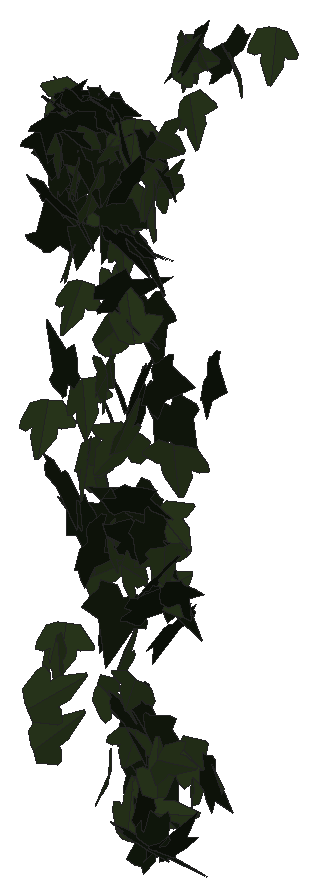
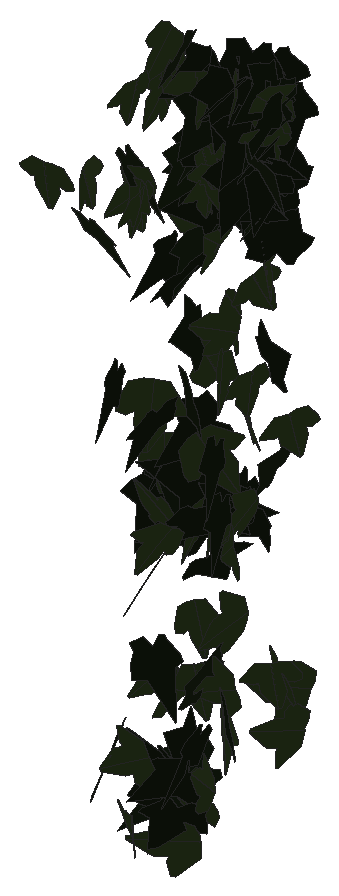
# SketchUp Ruby script. Lengths in inches.
U = 1.inch
M = Sketchup.active_model
def pt(a) = Geom::Point3d.new(a.map { |v| v * U })
def face(e, loops, mat)
  f = e.add_face(loops[0].map { |a| pt(a) })
  loops[1..].each { |l| e.add_face(l.map { |a| pt(a) }).erase! }
  f.material = f.back_material = mat if mat
  f
end
# faces: each face lists its corners as indices into pts; further lists are holes
def faces(e, pts, list, mat = nil) = list.each { |f| face(e, (f[0].is_a?(Array) ? f : [f]).map { |l| l.map { |i| pts[i] } }, mat) }
# xy, xz, yz: faces in a plane at the given z, y or x. An outline is a flat list of corners, or four numbers for a rectangle; further outlines are holes
def ring(l) = l.size == 4 ? [[l[0], l[1]], [l[2], l[1]], [l[2], l[3]], [l[0], l[3]]] : l.each_slice(2).to_a
def flat(e, list, mat, &to3) = list.each { |f| face(e, (f[0].is_a?(Array) ? f : [f]).map { |l| ring(l).map { |u, v| to3.(u, v) } }, mat) }
def xy(e, z, list, mat = nil) = flat(e, list, mat) { |x, y| [x, y, z] }
def xz(e, y, list, mat = nil) = flat(e, list, mat) { |x, z| [x, y, z] }
def yz(e, x, list, mat = nil) = flat(e, list, mat) { |y, z| [x, y, z] }
def lines(e, pts, list) = list.each { |a, b| e.add_line(pt(pts[a]), pt(pts[b])) }
# prism: a flat outline (further loops are holes) pulled along v
def prism(e, loops, v, mat = nil)
  f = face(e, loops, mat); d = Geom::Vector3d.new(v.map { |x| x * U })
  f.pushpull(f.normal.samedirection?(d) ? d.length : -d.length)
end
def box(e, o, s, mat = nil) = prism(e, [[o, [o[0] + s[0], o[1], o[2]], [o[0] + s[0], o[1] + s[1], o[2]], [o[0], o[1] + s[1], o[2]]]], [0, 0, s[2]], mat)
def at(x, y, z, deg = 0) = Geom::Transformation.translation(pt([x, y, z])) * Geom::Transformation.rotation(ORIGIN, Z_AXIS, deg.degrees)
def axes(o, x, y, z) = Geom::Transformation.new([*x, 0, *y, 0, *z, 0, *pt(o).to_a, 1])
def part(name) = M.definitions.add(name)
# library, detail: a bought-in or finely detailed component or shape, given as its bounding box
def library(name, o, s) = part(name).tap { |d| box(d.entities, o, s) }
def detail(e, o, s) = box(e.add_group.entities, o, s)
def put(e, d, t, mat = nil) = e.add_instance(d, t).tap { |i| i.material = mat if mat }
def group(e, t, mat = nil) = e.add_group.tap { |g| g.transformation = t; g.material = mat if mat }.entities
root = M.entities
M.materials.add("efeu1").color = [18, 25, 13]
M.materials.add("efeu2").color = [43, 57, 29]
c1 = part("ivyleaf_10")
p = [[0,0.5,-0.03],[-0.0625,2.02,-0.43],[-0.19,2.01,-0.46],[-0.54,1.05,-0.29],[-0.52,0.625,-0.18],[-0.83,0.76,-0.28],
  [-1.16,0.64,-0.33],[-1.15,0.33,-0.24],[-0.77,-0.39,0.02],[-0.3,-0.51,0.16],[0.04,-0.48,0.23],[-0.02,2.01,-0.4375],
  [-0.06,2.01,-0.43],[0.04,-0.49,0.23],[0.67,-0.49,0.14],[1.38,0.36,-0.2],[1.375,0.51,-0.24],[0.81,0.65,-0.19],
  [0.62,0.59,-0.15],[0.6,1.09,-0.28],[0.5,1.23,-0.31]]
faces(c1.entities,p,[[0,1,2,3,4,5,6,7,8,9,10],[11,12,0,13,14,15,16,17,18,19,20]],"efeu2")
c2 = part("ivyleaf_9")
p = [[1.54,2.16,1.25],[1.36,2.04,1.19],[-0.21,0.99,0.68],[-0.71,1.11,0.82],[-0.85,0.86,0.67],[-0.8,0.17,0.21],
  [-0.9,-0.01,0.1],[-0.67,-0.16,-0.02],[-0.08,-0.08,-0.05],[-0.03,-0.6,-0.4],[0.65,-0.88,-0.66],[0.83,-0.6,-0.49],
  [1.29,-0.42,-0.43],[1.8125,-0.07,-0.26],[1.21,0.44,0.15]]
faces(c2.entities,p,[[0,1,2,3,4,5,6,7,8,9,10,11,12,13,14]],"efeu1")
put(root,c1,axes([585.52,128.9,222.65],[-0.54212,-0.81235,-0.06265],[0.0387,0.04949,-0.97662],[0.81384,-0.54348,0.00471]))
put(root,c1,axes([578.94,128.14,213.07],[0.2301,0.27895,-1.14359],[0.75107,0.86242,0.36148],[0.90636,-0.78547,-0.00923]))
put(root,c2,axes([585.55,128.49,221.7],[-0.16843,0.93935,0.08399],[-0.01678,0.08232,-0.95433],[-0.94295,-0.16925,0.00198]))
put(root,c1,axes([583.87,128.9,215.3125],[-0.8398,-0.13492,0.40747],[-0.40406,-0.05358,-0.85051],[0.14482,-0.9319,-0.01009]))
put(root,c1,axes([584.26,129.4,240.45],[0.591,-0.3393,0.87922],[0.78325,-0.40029,-0.68097],[0.52408,0.98085,0.02624]))
put(root,c1,axes([583.77,128.875,233.49],[1.03176,0.22803,0.28353],[-0.27668,-0.06193,1.05665],[0.23628,-1.06821,-0.00074]))
put(root,c1,axes([580.61,129.42,225.9375],[0.68534,-0.54383,0.62493],[0.48946,-0.38853,-0.8749],[0.66836,0.84218,-0.00008]))
put(root,c2,axes([585.53,128.27,231.74],[0.19674,0.06037,-0.97596],[-0.53263,0.84148,-0.05532],[0.82003,0.53208,0.19823]))
put(root,c1,axes([582.47,128.65,210.42],[0.258,-0.77552,-0.70588],[-0.26578,0.65484,-0.81659],[1.01443,0.36881,-0.03442]))
put(root,c1,axes([579.13,128.17,211.02],[0.13674,0.28511,-1.14107],[0.52764,1.0118,0.31605],[1.05116,-0.54497,-0.0102]))
put(root,c2,axes([579.0625,129.56,224.1],[0.38561,-0.86651,0.45505],[0.21061,-0.40417,-0.9481],[0.9558,0.43864,0.02533]))
put(root,c1,axes([582.14,128.72,230.53],[0.60013,-0.50816,-0.7164],[-0.37655,0.63502,-0.76587],[0.79351,0.68566,0.17838]))
put(root,c2,axes([579.81,128.97,242.88],[0.24566,0.88942,-0.62998],[-0.19521,-0.59944,-0.92242],[-1.07231,0.31289,0.0236]))
put(root,c2,axes([582.44,129.68,218.75],[-0.31214,-1.02487,0.06024],[-0.01116,-0.05958,-1.07133],[1.02658,-0.31227,0.00667]))
put(root,c2,axes([582.68,128.41,234.93],[0.42243,0.24262,0.96228],[0.78221,0.56223,-0.48513],[-0.61074,0.88788,0.04424]))
put(root,c2,axes([583.09,128.75,238.09],[0.98483,0.26717,-0.34487],[-0.34553,-0.0421,-1.01933],[-0.26631,1.04262,0.04721]))
put(root,c2,axes([584.45,128.92,223.63],[0.54954,-0.67759,-0.64036],[-0.36194,0.52997,-0.87139],[0.85918,0.65665,0.0425]))
put(root,c1,axes([585.16,128.76,210.67],[0.07017,0.97933,-0.387],[-0.00979,0.38845,0.98122],[1.05298,-0.06165,0.03491]))
put(root,c1,axes([583.65,128.98,212.43],[0.85574,0.31412,-0.23921],[-0.34595,0.32134,-0.81563],[-0.19029,0.82841,0.40709]))
put(root,c1,axes([580.97,129.32,238.61],[0.13724,-1.08276,-0.04315],[0.03719,-0.03876,1.09095],[-1.08298,-0.13854,0.03199]))
put(root,c2,axes([584.12,128.51,219.38],[0.54084,0.38582,0.68539],[0.51903,0.44988,-0.66282],[-0.59095,0.74824,0.04511]))
put(root,c2,axes([581.52,128.47,221.9],[0.14842,-0.06138,-1.12897],[-0.78639,0.81252,-0.14756],[0.81236,0.79776,0.06342]))
put(root,c1,axes([582.93,129,227.37],[0.25347,-0.95085,0.36997],[-0.07167,0.36368,0.98378],[-1.01777,-0.26241,0.02287]))
put(root,c1,axes([580.34,129.04,240.625],[0.51319,-0.83155,-0.41195],[-0.09299,0.4223,-0.96828],[0.92332,0.50471,0.13145]))
put(root,c2,axes([585.04,128.85,207.48],[-0.86174,0.08361,-0.60119],[-0.59853,0.05649,0.86579],[0.1009,1.04921,0.0013]))
put(root,c1,axes([584.46,129.84,241.3],[0.17698,-0.79659,0.68255],[0.3458,-0.6092,-0.80066],[0.99038,0.35506,0.15759]))
put(root,c2,axes([583.84,128.58,207.7],[1.45844,-0.06622,-0.10201],[-0.07329,0.5011,-1.37309],[0.09706,1.37345,0.49605]))
put(root,c2,axes([579.14,129.06,241.66],[0.53688,0.79531,-0.56534],[-0.31461,-0.46971,-0.95956],[-0.92366,0.62227,-0.00176]))
put(root,c1,axes([585.58,128.85,212.04],[-0.26101,-0.39466,-0.79136],[0.44292,0.65581,-0.47315],[0.7654,-0.51409,0.00393]))
put(root,c2,axes([583.01,128.83,224.63],[0.8427,0.49196,0.32927],[0.29036,0.15569,-0.97572],[-0.51588,0.89125,-0.01131]))
put(root,c2,axes([583.47,128.53,241.17],[-0.21376,0.56597,-0.88787],[-0.3776,0.80452,0.60374],[0.98288,0.43217,0.03884]))
put(root,c2,axes([582.53,130.01,212.86],[0.33744,-0.86068,0.59164],[0.3391,-0.49778,-0.91755],[0.98783,0.46488,0.11287]))
put(root,c1,axes([579,129.68,241.5],[0.29646,-0.93548,0.17038],[0.23257,-0.10171,-0.96313],[0.92199,0.32646,0.18817]))
put(root,c2,axes([579.89,129.73,241.35],[0.49213,-0.9195,-0.04882],[-0.02424,0.0424,-1.04291],[0.92047,0.49272,-0.00136]))
put(root,c2,axes([583.23,129.73,237.63],[0.61706,-0.77703,0.18831],[0.13739,-0.13128,-0.99191],[0.78763,0.63166,0.0255]))
put(root,c2,axes([585.39,129.06,220.6875],[0.74433,0.61958,-0.12804],[-0.08391,-0.09929,-0.9682],[-0.62709,0.74871,-0.02243]))
put(root,c2,axes([582.78,129.4,222.02],[0.54904,-0.15476,0.95297],[0.94806,-0.12076,-0.56582],[0.18246,1.09317,0.0724]))
put(root,c2,axes([577.85,129.79,237.98],[0.52872,-0.4296,0.7182],[0.60121,-0.39598,-0.67945],[0.58217,0.7991,0.04941]))
put(root,c2,axes([584.97,129.41,206.8],[0.46852,0.91791,0.16625],[-0.09763,-0.13677,1.03028],[0.92772,-0.47796,0.02446]))
put(root,c1,axes([578.03,129.78,226.87],[0.54704,0.86913,-0.2398],[-0.13372,-0.19917,-1.02694],[-0.89163,0.5631,0.00689]))
put(root,c1,axes([578.37,130.04,214.75],[0.7305,-0.29535,0.69025],[0.63552,-0.26951,-0.7879],[0.39974,0.96822,-0.00876]))
put(root,c2,axes([584.11,129.1,208.58],[0.018,-0.22074,1.05801],[0.32906,1.00904,0.20492],[-1.02948,0.31867,0.084]))
put(root,c1,axes([579.86,129.73,241.99],[-0.93456,-0.22475,0.28094],[-0.27652,-0.05155,-0.9611],[0.23016,-0.97451,-0.01395]))
put(root,c1,axes([584.54,129.98,219.93],[0.62137,-0.23138,-0.81582],[0.78794,-0.21628,0.66148],[-0.31342,-1.00243,0.04559]))
put(root,c2,axes([583.14,129.29,233.71],[0.78131,0.34884,-0.6272],[-0.71739,0.35315,-0.69724],[-0.02048,0.93761,0.49596]))
put(root,c2,axes([579.62,130.18,222.32],[-0.39694,-0.04592,-0.95874],[0.94327,0.17331,-0.39883],[0.1776,-1.02309,-0.02453]))
put(root,c2,axes([579.37,129.5625,229.09],[0.0552,0.013,1.05977],[-0.5311,0.91869,0.01639],[-0.91718,-0.5312,0.05429]))
put(root,c2,axes([580.15,129.73,243.48],[0.74838,0.43766,-0.76082],[-0.68377,-0.33618,-0.86598],[-0.55033,1.01287,0.04132]))
put(root,c2,axes([583.04,129.33,237.51],[1.0056,0.36089,-0.16373],[-0.29156,0.3713,-0.97233],[-0.26841,0.94878,0.44279]))
put(root,c2,axes([583.57,130.3,242.5],[0.59373,-0.82559,0.0581],[0.02891,-0.05077,-1.0169],[0.82712,0.59441,-0.00616]))
put(root,c1,axes([579.46,130.33,233.27],[0.33452,0.81783,-0.44955],[-0.2388,-0.38665,-0.88109],[-0.90218,0.40559,0.06653]))
put(root,c1,axes([582.11,130.15,237.01],[0.08343,0.99386,-0.10781],[-0.01299,-0.1071,-0.99735],[-0.9996,0.08434,0.00397]))
put(root,c1,axes([579.9,130.18,228.4],[0.1988,1.03837,-0.09617],[-0.01793,-0.09448,-1.05723],[-1.04266,0.19961,-0.00016]))
put(root,c2,axes([581.85,130.65,238.63],[-0.71991,-0.68236,-0.17883],[0.11771,0.13572,-0.99175],[0.69551,-0.72926,-0.01725]))
put(root,c2,axes([581.47,130.14,221.74],[-0.32575,0.15785,1.01209],[-0.9123,0.43823,-0.36197],[-0.46578,-0.96871,0.00117]))
put(root,c2,axes([578.2,130.54,235.29],[0.78771,0.20273,0.63781],[-0.63522,-0.08367,0.8111],[0.21071,-1.01009,0.06083]))
put(root,c1,axes([580.96,130.3,213.24],[0.38495,-0.06136,0.95296],[0.94684,0.15797,-0.37231],[-0.12402,1.01556,0.11549]))
put(root,c1,axes([582.92,129.625,220.59],[-0.24828,0.62545,0.83654],[-0.36423,0.75403,-0.67186],[-0.97894,-0.43918,0.03781]))
put(root,c1,axes([582.54,130.19,206.96],[1.13403,-0.11412,0.10794],[-0.10741,0.01072,1.13975],[-0.11463,-1.1391,-0.00008]))
put(root,c1,axes([579.61,130.5,240.43],[-0.83811,-0.65835,0.06001],[-0.0405,-0.04559,-1.06571],[0.65984,-0.83902,0.01081]))
put(root,c1,axes([581.78,129.9,221.51],[-0.36671,0.6527,0.75917],[-0.4522,0.61334,-0.74575],[-0.89323,-0.57846,0.06587]))
put(root,c2,axes([581.11,130.89,242.29],[0.13969,-0.07753,-0.99855],[0.99934,-0.05626,0.14416],[-0.0666,-1.0067,0.06884]))
put(root,c1,axes([584.44,130.01,242.95],[-0.19559,-0.71341,-0.80037],[0.18191,0.7797,-0.73944],[1.05662,-0.26629,-0.02085]))
put(root,c1,axes([578.36,130.63,215.2],[0.78528,0.64052,-0.09761],[-0.07543,-0.06196,-1.01338],[-0.64351,0.78889,-0.00034]))
put(root,c2,axes([580.72,131.11,241.02],[-0.28691,-0.95809,-0.03676],[0.0429,0.0255,-0.99956],[0.95784,-0.28813,0.03376]))
put(root,c1,axes([578.22,131.27,242.61],[-0.4296,-0.52454,0.73994],[0.04439,-0.82993,-0.56256],[0.90592,-0.20808,0.37846]))
put(root,c1,axes([578.84,130.55,235.07],[0.47019,-0.86818,-0.31057],[-0.11266,0.29192,-0.98659],[0.91515,0.48199,0.03811]))
put(root,c1,axes([581.21,130.69,237.85],[0.93812,0.34984,-0.01559],[-0.0324,0.04231,-0.99993],[-0.34868,0.9373,0.05095]))
put(root,c2,axes([582.97,129.85,229.22],[0.12675,0.21286,1.05108],[0.17479,1.04015,-0.23172],[-1.05808,0.19732,0.08764]))
put(root,c1,axes([581.72,130,234.1],[0.15099,0.60151,-0.79965],[-0.03363,0.81129,0.60392],[1.00006,-0.06354,0.14104]))
put(root,c2,axes([577.9,130.55,242.29],[0.87475,-0.32857,0.32868],[0.38241,0.11076,-0.90701],[0.26411,0.92787,0.22466]))
put(root,c1,axes([578.375,130.97,242.04],[0.99941,-0.12496,0.14333],[0.14086,-0.02865,-1.00714],[0.12775,1.00923,-0.01084]))
put(root,c1,axes([581.92,130.84,239.2],[0.97935,0.01814,-0.22956],[-0.22841,0.20366,-0.95838],[0.02919,0.98506,0.20237]))
put(root,c2,axes([578.48,130.0625,242.61],[0.38369,0.61781,0.68585],[0.2866,0.62631,-0.72451],[-0.87747,0.47472,0.06327]))
put(root,c1,axes([584.55,130.17,240.5],[0.11173,0.42951,0.91597],[-0.41757,0.85895,-0.35183],[-0.92147,-0.33716,0.2705]))
put(root,c2,axes([579.22,131.32,237.24],[-0.62628,-0.69699,-0.34339],[0.22583,0.25873,-0.93701],[0.74344,-0.66573,-0.00464]))
put(root,c2,axes([580.55,131.37,240.39],[-0.9853,-0.15087,-0.10176],[0.10198,0.00626,-0.99674],[0.15072,-0.99052,0.0092]))
put(root,c2,axes([578.05,131.46,239.83],[-0.7576,-0.555,-0.33157],[0.32507,0.1145,-0.93442],[0.55883,-0.81902,0.09405]))
put(root,c1,axes([579.61,131.63,242.5625],[-0.18743,0.4667,-0.86016],[0.23021,-0.83019,-0.5006],[-0.95115,-0.2929,0.04834]))
put(root,c1,axes([581.29,131.11,241.37],[-0.0535,-1.00265,-0.12054],[0.00289,0.12056,-1.00407],[1.00987,-0.05347,-0.00351]))
put(root,c2,axes([578.24,131.63,240.1],[0.12981,-0.96576,0.16948],[-0.00079,-0.17106,-0.97416],[0.98051,0.12772,-0.02322]))
put(root,c1,axes([584.48,131.07,226.43],[-1.16472,-0.38803,0.0493],[-0.04499,-0.02094,-1.22765],[0.38855,-1.16558,0.00564]))
put(root,c1,axes([582.03,131.05,242.17],[0.79875,0.62419,-0.04644],[-0.17079,0.14492,-0.98975],[-0.60216,0.78687,0.21912]))
put(root,c2,axes([578.16,131.51,237.54],[0.4645,-0.87812,0.05848],[0.04485,-0.04242,-0.99321],[0.87892,0.46625,0.01978]))
put(root,c2,axes([582.41,131.64,233.15],[0.19807,-1.07852,-0.14883],[-0.02996,0.14582,-1.09655],[1.08833,0.2003,-0.0031]))
put(root,c2,axes([578.29,131.01,239.35],[0.73858,0.50277,-0.43038],[-0.38435,-0.19917,-0.89225],[-0.53878,0.8313,0.04652]))
put(root,c1,axes([578.21,131.55,241.07],[0.64787,0.7063,-0.25248],[-0.22463,-0.13561,-0.95577],[-0.71565,0.68197,0.07144]))
put(root,c2,axes([578.16,131.12,242.68],[0.90573,0.04013,-0.61368],[-0.61482,0.08494,-0.90186],[0.01456,1.09075,0.09281]))
put(root,c2,axes([579.875,131.93,242.55],[0.20425,-0.97394,0.04392],[0.09018,-0.02581,-0.99167],[0.97075,0.20731,0.08288]))
put(root,c1,axes([580.95,131.95,225.57],[-0.73032,-0.6283,0.73122],[-0.5142,-0.52211,-0.96219],[0.8155,-0.89188,0.04815]))
put(root,c1,axes([580.36,131.34,229.5],[0.24415,-0.88004,-0.54564],[-0.03826,0.55255,-0.90831],[1.03476,0.22808,0.09515]))
put(root,c2,axes([580.01,131.29,242.81],[0.72241,0.60815,-0.343],[-0.30347,-0.17102,-0.94235],[-0.62881,0.7812,0.06073]))
put(root,c1,axes([580.45,131.07,230.85],[0.02049,-0.48905,0.90607],[0.01743,0.90628,0.48877],[-1.02948,0.00561,0.02631]))
put(root,c2,axes([578.47,131.41,240.13],[-0.5169,0.80965,0.27333],[-0.14708,0.23038,-0.96058],[-0.84178,-0.53742,0]))
put(root,c2,axes([583.59,131.61,219.05],[0.66478,-0.6276,-0.5162],[-0.32917,0.40178,-0.91242],[0.74296,0.73957,0.05763]))
put(root,c2,axes([581.07,131.16,241.12],[0.50588,0.77261,0.4094],[0.00793,0.46891,-0.89471],[-0.87434,0.45127,0.22877]))
put(root,c2,axes([579.23,131.39,238.9],[0.5287,0.8494,0.01435],[-0.06528,0.05747,-0.99682],[-0.84701,0.52577,0.08578]))
put(root,c2,axes([581.67,132.5,221.81],[-0.3833,-0.83198,-0.45171],[-0.15058,-0.42754,0.91525],[-0.93464,0.41008,0.03779]))
put(root,c2,axes([578.61,131.53,241.24],[0.55897,0.80506,0.1598],[0.11097,0.11744,-0.9798],[-0.81323,0.56938,-0.02385]))
put(root,c2,axes([585.61,131.8,210.14],[0.61921,-0.34894,-0.75473],[-0.62039,0.43266,-0.70903],[0.55362,0.87512,0.04961]))
put(root,c2,axes([581.94,131.49,227.12],[0.01453,0.29885,1.02923],[-0.17623,1.01598,-0.29251],[-1.05715,-0.16526,0.06291]))
put(root,c1,axes([581.71,132.27,206.58],[0.0241,-0.14888,-1.18285],[1.1396,0.35037,-0.02088],[0.35016,-1.13003,0.14937]))
put(root,c1,axes([578.63,131.91,223.45],[-0.14181,0.44389,0.94563],[-0.23281,0.91687,-0.46531],[-1.01836,-0.27142,-0.02531]))
put(root,c1,axes([583.77,132.63,209.99],[0.51872,0.05072,1.0102],[0.9709,0.29336,-0.51327],[-0.28361,1.09705,0.09055]))
put(root,c2,axes([581.04,132.2,211.74],[0.43572,-0.27691,-0.99762],[-0.67211,0.74764,-0.50107],[0.78752,0.79128,0.12432]))
put(root,c1,axes([579.26,131.94,217.93],[0.03088,0.11792,1.18277],[-0.25354,1.15659,-0.10869],[-1.16128,-0.24938,0.05519]))
put(root,c2,axes([581.65,132.85,208.42],[-0.24012,-0.6266,-0.77616],[0.31762,0.70876,-0.67045],[0.94561,-0.39718,0.0281]))
put(root,c2,axes([581.27,132.75,210.24],[0.16587,-0.30042,-0.96853],[0.38755,0.92568,-0.22076],[0.93707,-0.32966,0.26274]))
put(root,c1,axes([578.05,133.66,222.43],[0.49067,-0.38603,0.86918],[0.82687,-0.31005,-0.60449],[0.46987,0.94874,0.15611]))
put(root,c2,axes([582.51,133.22,227.06],[0.35273,-0.84193,-0.60469],[-0.25644,0.54801,-0.91261],[1.00436,0.43561,-0.02065]))
put(root,c2,axes([582.5,133.33,215.93],[-0.31724,0.97874,-0.31163],[0.10082,-0.29491,-1.02886],[-1.02219,-0.33284,-0.00476]))
put(root,c1,axes([582.16,133.04,221.37],[0.29579,0.80071,0.57967],[0.22845,0.53331,-0.85325],[-0.96175,0.37294,-0.0244]))
put(root,c1,axes([583.24,133.72,242.69],[0.06896,1.00786,-0.02215],[0.00357,-0.02245,-1.01021],[-1.0081,0.06886,-0.00509]))
put(root,c2,axes([578.94,133.71,226.86],[0.57911,0.00624,-0.82687],[-0.82118,0.12282,-0.5742],[0.09705,1.002,0.07554]))
put(root,c1,axes([583.19,134.02,207.2],[0.71885,-0.43025,0.61389],[-0.52552,0.31731,0.83776],[-0.5346,-0.89045,0.00192]))
put(root,c2,axes([578.29,133.63,213.89],[-0.02265,0.18044,1.03554],[-0.16094,1.02297,-0.18177],[-1.03875,-0.16244,0.00558]))
put(root,c2,axes([583.93,134.09,228.84],[0.19766,-0.11246,-1.01213],[-0.81732,0.59753,-0.22601],[0.6075,0.8405,0.02525]))
put(root,c2,axes([578.18,134.27,224.68],[0.56445,0.06045,-0.83067],[-0.82818,0.14705,-0.55206],[0.08824,0.99348,0.13226]))
put(root,c1,axes([578.11,135.25,211.66],[0.3864,-0.63857,0.67365],[-0.32533,0.59023,0.7461],[-0.86933,-0.50471,0.02021]))
put(root,c2,axes([579.77,138.43,242.51],[-0.75391,0.68328,-0.16283],[0.12523,-0.10429,-1.01745],[-0.69116,-0.76421,-0.00674]))
put(root,c1,axes([579.04,138.41,241.41],[0.15664,0.25276,0.98298],[0.00619,0.99436,-0.25667],[-1.01493,0.04508,0.15014]))
put(root,c1,axes([578.39,139.45,241.52],[-0.02037,0.94308,-0.29113],[-0.06062,-0.29184,-0.94114],[-0.98514,-0.00155,0.06393]))
put(root,c1,axes([578.69,139.26,241.7],[-0.91436,0.36362,0.11866],[-0.12606,0.00381,-0.98308],[-0.36112,-0.92202,0.04274]))
put(root,c1,axes([581.39,139.16,241.44],[0.34245,0.0888,-0.96523],[-0.5568,0.85597,-0.11879],[0.79342,0.56237,0.33323]))
put(root,c1,axes([581.98,141.125,242.39],[1.01966,0.0885,0.10843],[0.10881,0.00034,-1.02345],[-0.08804,1.02541,-0.00902]))
put(root,c2,axes([579.57,141.16,240.66],[-0.59873,0.74006,0.36971],[-0.34991,0.187,-0.94098],[-0.74963,-0.67838,0.14394]))
